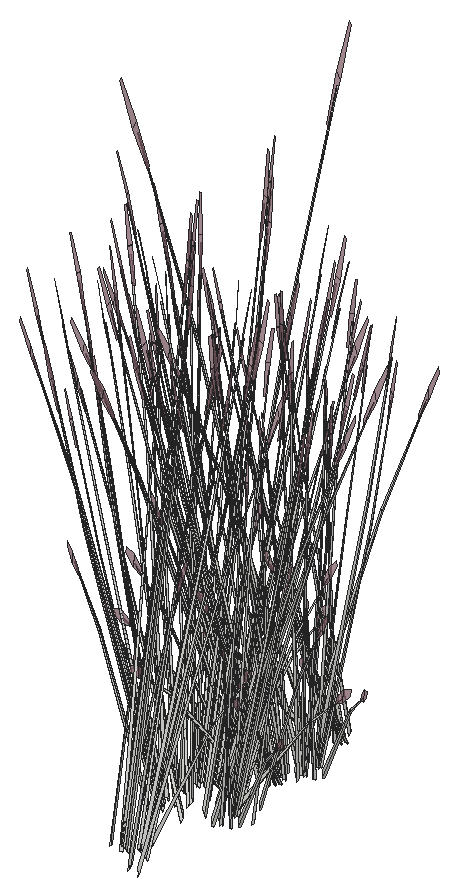
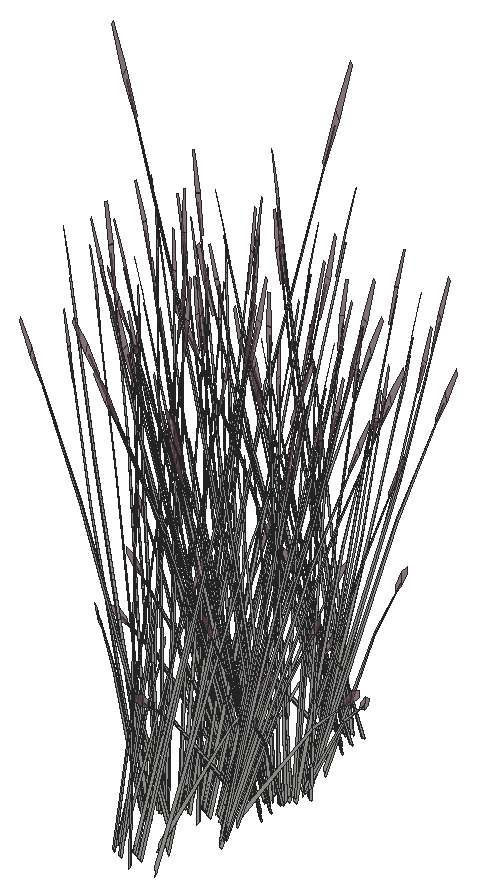
# SketchUp Ruby script. Lengths in inches.
U = 1.inch
M = Sketchup.active_model
def pt(a) = Geom::Point3d.new(a.map { |v| v * U })
def face(e, loops, mat)
  f = e.add_face(loops[0].map { |a| pt(a) })
  loops[1..].each { |l| e.add_face(l.map { |a| pt(a) }).erase! }
  f.material = f.back_material = mat if mat
  f
end
# faces: each face lists its corners as indices into pts; further lists are holes
def faces(e, pts, list, mat = nil) = list.each { |f| face(e, (f[0].is_a?(Array) ? f : [f]).map { |l| l.map { |i| pts[i] } }, mat) }
# xy, xz, yz: faces in a plane at the given z, y or x. An outline is a flat list of corners, or four numbers for a rectangle; further outlines are holes
def ring(l) = l.size == 4 ? [[l[0], l[1]], [l[2], l[1]], [l[2], l[3]], [l[0], l[3]]] : l.each_slice(2).to_a
def flat(e, list, mat, &to3) = list.each { |f| face(e, (f[0].is_a?(Array) ? f : [f]).map { |l| ring(l).map { |u, v| to3.(u, v) } }, mat) }
def xy(e, z, list, mat = nil) = flat(e, list, mat) { |x, y| [x, y, z] }
def xz(e, y, list, mat = nil) = flat(e, list, mat) { |x, z| [x, y, z] }
def yz(e, x, list, mat = nil) = flat(e, list, mat) { |y, z| [x, y, z] }
def lines(e, pts, list) = list.each { |a, b| e.add_line(pt(pts[a]), pt(pts[b])) }
# prism: a flat outline (further loops are holes) pulled along v
def prism(e, loops, v, mat = nil)
  f = face(e, loops, mat); d = Geom::Vector3d.new(v.map { |x| x * U })
  f.pushpull(f.normal.samedirection?(d) ? d.length : -d.length)
end
def box(e, o, s, mat = nil) = prism(e, [[o, [o[0] + s[0], o[1], o[2]], [o[0] + s[0], o[1] + s[1], o[2]], [o[0], o[1] + s[1], o[2]]]], [0, 0, s[2]], mat)
def at(x, y, z, deg = 0) = Geom::Transformation.translation(pt([x, y, z])) * Geom::Transformation.rotation(ORIGIN, Z_AXIS, deg.degrees)
def axes(o, x, y, z) = Geom::Transformation.new([*x, 0, *y, 0, *z, 0, *pt(o).to_a, 1])
def part(name) = M.definitions.add(name)
# library, detail: a bought-in or finely detailed component or shape, given as its bounding box
def library(name, o, s) = part(name).tap { |d| box(d.entities, o, s) }
def detail(e, o, s) = box(e.add_group.entities, o, s)
def put(e, d, t, mat = nil) = e.add_instance(d, t).tap { |i| i.material = mat if mat }
def group(e, t, mat = nil) = e.add_group.tap { |g| g.transformation = t; g.material = mat if mat }.entities
root = M.entities
M.materials.add("LightPink_Translucent").color = [144, 107, 117]
M.materials["LightPink_Translucent"].alpha = 0.75
c1 = part("blade")
p = [[2.15,0.21,22],[0,0.17,0],[0.09,0.45,0],[2.18,0.31,22],[2.29,0.31,22],[0.38,0.45,0],
  [2.48,0.24,33],[2.49,0.24,33],[2.48,0.22,33]]
faces(c1.entities,p,[[0,1,2,3],[4,5,2,3],[6,3,4,7],[8,0,3,6]])
c2 = part("seeds")
p = [[0.3,-0.1,1.38],[-0.01,-0.03,1.59],[-0.01,-0.03,0.03],[0.14,-0.07,-0.07],[0.29,-0.03,3],[0.15,0.01,3.11]]
faces(c2.entities,p,[[0,1,2,3],[1,0,4,5]],"LightPink_Translucent")
c3 = part("blade with seeds")
put(c3.entities,c1,at(0,0,0))
put(c3.entities,c2,axes([2.4,0.25,30.99],[1.5799,-0.05474,1.17369],[-0.12525,1.92788,0.29478],[-0.07173,-0.02425,1.56792]))
put(root,c3,axes([429.37,403.85,153.98],[-0.05353,-0.00358,1.49853],[-0.22227,-0.38383,-0.1416],[0.08926,-0.1262,0.26519]))
put(root,c3,axes([427.31,399,154],[-0.30197,0.1603,0.05432],[-0.1478,-0.29231,0.42765],[0.02916,0.12885,0.65209]))
put(root,c3,axes([426.5,398.62,153.82],[-0.27728,0.24833,-0.29918],[-0.26248,-0.28355,0.38624],[-0.03994,0.14407,0.73904]))
put(root,c3,axes([425.54,398.54,153.98],[-0.01019,0.09334,1.47793],[0.28908,0.3247,-0.23373],[-0.07568,0.15355,0.11853]))
put(root,c3,axes([426.47,398.33,154.56],[0.45039,0.02337,-0.11403],[-0.01231,0.44247,-0.63292],[-0.03129,0.17041,0.9617]))
put(root,c3,axes([427.3,398.83,154.25],[0.40102,-0.2196,-0.10273],[0.19707,0.38974,-0.57019],[0.05291,0.16424,0.8664]))
put(root,c3,axes([428.54,403.7,153.82],[0.35672,-0.06741,-0.29918],[0.09419,0.38534,0.38624],[0.10222,-0.1035,0.73904]))
put(root,c3,axes([425.19,403.06,154],[0.02064,-0.35866,0.05432],[0.3116,0.00983,0.42765],[-0.11936,-0.03753,0.65209]))
put(root,c3,axes([425.07,403.17,153.82],[-0.23317,-0.29531,-0.29918],[0.26625,-0.27955,0.38624],[-0.13527,-0.04253,0.73904]))
put(root,c3,axes([426.77,398.5,154.23],[0.29336,0.31691,-0.47917],[-0.3099,0.27755,-0.37115],[-0.04464,0.16102,0.91684]))
put(root,c3,axes([427.64,398.81,153.95],[0.40284,0.11824,-0.43168],[-0.13808,0.40538,-0.33437],[0.03694,0.16321,0.82598]))
put(root,c3,axes([427.87,397.97,153.27],[-0.09368,-0.15143,1.44779],[0.43286,-0.12749,0.11706],[0.09783,0.23774,0.61892]))
put(root,c3,axes([427.46,399.06,153.82],[-0.12355,0.36271,-0.29918],[-0.36044,-0.10579,0.38624],[0.03305,0.14603,0.73904]))
put(root,c3,axes([426.68,398.36,154.51],[-0.01066,0.43628,-0.66621],[-0.44902,-0.0293,0.0804],[-0.04739,0.18483,0.94242]))
put(root,c3,axes([425.32,403.37,154.21],[-0.40965,-0.01136,-0.60019],[0.02751,-0.47821,0.07243],[-0.17355,-0.05047,0.84903]))
put(root,c3,axes([425.51,399.5,153.98],[0.04649,-0.02848,1.49853],[0.38427,0.18941,-0.1416],[-0.00903,0.15771,0.26519]))
put(root,c3,axes([427.11,398.05,153.27],[-0.01003,-0.18103,1.44779],[0.43473,0.12009,0.11706],[-0.02689,0.25798,0.61892]))
put(root,c3,axes([428.57,403.87,154],[0.28133,0.19836,0.05432],[-0.16379,0.28248,0.42765],[0.0902,-0.09132,0.65209]))
put(root,c3,axes([429.57,404.31,153.98],[0.05687,-0.07184,1.47793],[-0.07279,-0.44069,-0.23373],[0.14268,-0.08356,0.11853]))
put(root,c3,axes([427.5,398.73,154.21],[0.19559,0.38351,-0.60019],[-0.40262,0.21373,0.07243],[0.04574,0.1853,0.84903]))
put(root,c3,axes([424.76,402.59,153.98],[0.03038,0.04707,1.49853],[-0.14646,0.42312,-0.1416],[-0.14833,0.00306,0.26519]))
put(root,c3,axes([427.2,399.7,153.98],[0.05195,0.07595,1.47793],[0.41921,0.02984,-0.23373],[0.04216,0.1675,0.11853]))
put(root,c3,axes([425.18,403.47,153.95],[-0.29757,0.31243,-0.43168],[-0.2606,-0.33005,-0.33437],[-0.15119,-0.04754,0.82598]))
put(root,c3,axes([425.34,403.14,154.25],[-0.02194,0.47967,-0.10273],[-0.41546,-0.01311,-0.57019],[-0.16001,-0.03332,0.8664]))
put(root,c3,axes([428.45,404.98,154.25],[-0.20619,-0.42709,-0.10273],[0.36595,-0.20988,-0.57019],[0.15422,-0.05635,0.8664]))
put(root,c3,axes([428.43,404.61,153.95],[0.11102,-0.42903,-0.43168],[0.38064,0.14706,-0.33437],[0.15325,-0.03934,0.82598]))
put(root,c3,axes([426.53,398.97,152.84],[0.009,-0.24349,1.30391],[0.40497,0.12861,0.18019],[-0.03509,0.2595,0.61571]))
put(root,c3,axes([424.81,403.8,153.27],[0.16998,-0.01068,1.44779],[-0.11276,0.46299,0.11706],[-0.24224,-0.02864,0.61892]))
put(root,c3,axes([428.36,404.77,154.21],[0.3601,-0.20831,-0.60019],[0.20068,0.4288,0.07243],[0.17399,-0.04871,0.84903]))
put(root,c3,axes([424.71,404.04,154],[-0.15051,-0.3216,0.05432],[0.27447,-0.15741,0.42765],[-0.12099,0.03106,0.65209]))
put(root,c3,axes([428.66,404.81,153.82],[0.34057,0.13158,-0.29918],[-0.09933,0.38387,0.38624],[0.13712,-0.0352,0.73904]))
put(root,c3,axes([424.66,404.2,153.82],[-0.34057,-0.13158,-0.29918],[0.09933,-0.38387,0.38624],[-0.13712,0.0352,0.73904]))
put(root,c3,axes([427.74,404.33,153.27],[-0.16998,0.01068,1.44779],[0.11276,-0.46299,0.11706],[0.24224,0.02864,0.61892]))
put(root,c3,axes([428.61,404.97,154],[0.15051,0.3216,0.05432],[-0.27447,0.15741,0.42765],[0.12099,-0.03106,0.65209]))
put(root,c3,axes([425.9,409.13,153.27],[0.09368,0.15143,1.44779],[-0.43286,0.12749,0.11706],[-0.09783,-0.23774,0.61892]))
put(root,c3,axes([426.62,408.13,153.98],[-0.06268,-0.06613,1.47793],[-0.4183,0.04193,-0.23373],[-0.06676,-0.15817,0.11853]))
put(root,c3,axes([425.7,404.13,152.82],[0.11649,-0.06823,1.49584],[0.04017,0.47639,0.11706],[-0.25231,0.06321,0.53462]))
put(root,c3,axes([427.06,409.25,154.21],[-0.19559,-0.38351,-0.60019],[0.40262,-0.21373,0.07243],[-0.04574,-0.1853,0.84903]))
put(root,c3,axes([429.27,406.25,153.98],[-0.03706,-0.04129,1.49853],[0.08106,-0.44261,-0.1416],[0.14596,-0.02828,0.26519]))
put(root,c3,axes([427.87,409.62,154.21],[0.01066,-0.43628,-0.60019],[0.44902,0.0293,0.07243],[0.04739,-0.18483,0.84903]))
put(root,c3,axes([424.45,404.45,153.98],[-0.06692,0.06124,1.47793],[0.00569,0.44742,-0.23373],[-0.15339,0.05818,0.11853]))
put(root,c3,axes([424.89,404.39,153.95],[-0.11102,0.42903,-0.43168],[-0.38064,-0.14706,-0.33437],[-0.15325,0.03934,0.82598]))
put(root,c3,axes([424.875,404.03,154.25],[0.20619,0.42709,-0.10273],[-0.36595,0.20988,-0.57019],[-0.15422,0.05635,0.8664]))
put(root,c3,axes([428.95,405.88,153.32],[-0.07843,-0.39649,-0.0295],[0.37072,-0.09115,-0.13375],[0.07742,0.02514,0.44114]))
put(root,c3,axes([428.5,408.9375,153.98],[-0.00396,-0.09387,1.47793],[-0.33411,-0.2713,-0.23373],[0.05166,-0.16446,0.11853]))
put(root,c3,axes([427.09,408.92,153.82],[0.12355,-0.36271,-0.29918],[0.36044,0.10579,0.38624],[-0.03305,-0.14603,0.73904]))
put(root,c3,axes([427.37,409.4,153.27],[-0.0763,0.16212,1.44779],[-0.3201,-0.3355,0.11706],[0.1444,-0.2091,0.61892]))
put(root,c3,axes([427.98,405.87,154.25],[0.02194,-0.47967,-0.10273],[0.41546,0.01311,-0.57019],[0.16001,0.03332,0.8664]))
put(root,c3,axes([428.41,408.6,153.98],[-0.04162,0.03603,1.49853],[-0.40776,-0.12155,-0.1416],[-0.01476,-0.15722,0.26519]))
put(root,c3,axes([426.91,409.17,153.95],[-0.40284,-0.11824,-0.43168],[0.13808,-0.40538,-0.33437],[-0.03694,-0.16321,0.82598]))
put(root,c3,axes([427.78,409.48,153.95],[-0.29336,-0.31691,-0.43168],[0.3099,-0.27755,-0.33437],[0.04464,-0.16102,0.82598]))
put(root,c3,axes([426.1875,407.91,153.98],[-0.00765,0.05653,1.49853],[-0.37706,0.20517,-0.1416],[-0.11096,-0.10488,0.26519]))
put(root,c3,axes([428.35,405.58,153.98],[0.08791,-0.00798,1.47793],[0.24113,-0.36643,-0.23373],[0.15637,0.04837,0.11853]))
put(root,c3,axes([427.25,409.15,154.25],[-0.40102,0.2196,-0.10273],[-0.19707,-0.38974,-0.57019],[-0.05291,-0.16424,0.8664]))
put(root,c3,axes([428.09,409.64,154.25],[-0.45039,-0.02337,-0.10273],[0.01231,-0.44247,-0.57019],[0.03129,-0.17041,0.8664]))
put(root,c3,axes([424.75,405.14,154],[-0.28133,-0.19836,0.05432],[0.16379,-0.28248,0.42765],[-0.0902,0.09132,0.65209]))
put(root,c3,axes([428.06,409.36,153.82],[0.27728,-0.24833,-0.29918],[0.26248,0.28355,0.38624],[0.03994,-0.14407,0.73904]))
put(root,c3,axes([424.88,404.61,153.27],[0.14219,-0.09977,1.44779],[0.11971,0.461,0.11706],[-0.22323,0.10419,0.61892]))
put(root,c3,axes([427.25,408.97,154],[0.30197,-0.1603,0.05432],[0.1478,0.29231,0.42765],[-0.02916,-0.12885,0.65209]))
put(root,c3,axes([426.17,409.35,154.21],[-0.34944,-0.22798,-0.60019],[0.24834,-0.39949,0.07243],[-0.1266,-0.13612,0.84903]))
put(root,c3,axes([426.05,409.05,153.82],[-0.06329,-0.37991,-0.29918],[0.36182,-0.10032,0.38624],[-0.09718,-0.10887,0.73904]))
put(root,c3,axes([428.01,405.64,154.21],[0.40965,0.01136,-0.60019],[-0.02751,0.47821,0.07243],[0.17355,0.05047,0.84903]))
put(root,c3,axes([426.21,409.02,154],[0.18625,-0.29962,0.05432],[0.26523,0.17444,0.42765],[-0.08575,-0.09606,0.65209]))
put(root,c3,axes([423.7,404.9,153.98],[0.0523,0.01265,1.49853],[0.16179,0.41674,-0.1416],[-0.10706,0.10938,0.26519]))
put(root,c3,axes([425.28,409.6,153.27],[0.15222,0.08126,1.44779],[-0.31502,0.34091,0.11706],[-0.19634,-0.15379,0.61892]))
put(root,c3,axes([428.25,405.83,153.82],[0.23317,0.29531,-0.29918],[-0.26625,0.27955,0.38624],[0.13527,0.04253,0.73904]))
put(root,c3,axes([428.13,405.95,154],[-0.02064,0.35866,0.05432],[-0.3116,-0.00983,0.42765],[0.11936,0.03753,0.65209]))
put(root,c3,axes([424.78,405.3,153.82],[-0.35672,0.06741,-0.29918],[-0.09419,-0.38534,0.38624],[-0.10222,0.1035,0.73904]))
put(root,c3,axes([426.01,409.37,153.95],[-0.40438,0.11212,-0.43168],[-0.07074,-0.4246,-0.33437],[-0.10862,-0.12168,0.82598]))
put(root,c3,axes([426.29,408.99,154.59],[-0.2735,0.45217,-0.11506],[-0.39608,-0.2605,-0.63862],[-0.13768,-0.12775,0.97037]))
put(root,c3,axes([428.16,409.49,154],[0.33677,0.02198,0.05432],[-0.00923,0.33185,0.42765],[0.03524,-0.12712,0.65209]))
put(root,c3,axes([428.4,410.38,154.21],[0.21406,-0.37215,-0.60019],[0.37511,0.26448,0.07243],[0.12781,-0.13483,0.84903]))
put(root,c3,axes([428.39,410.21,153.95],[-0.10528,-0.43067,-0.43168],[0.39868,-0.07534,-0.33437],[0.11425,-0.11568,0.82598]))
put(root,c3,axes([427.41,405.08,153.27],[-0.15222,-0.08126,1.44779],[0.31502,-0.34091,0.11706],[0.19634,0.15379,0.61892]))
put(root,c3,axes([425.25,408.86,153.98],[-0.08817,-0.00333,1.47793],[-0.28072,0.33293,-0.23373],[-0.14978,-0.06803,0.11853]))
put(root,c3,axes([428.58,410.51,154.25],[-0.37908,-0.26007,-0.10273],[0.21839,-0.37663,-0.57019],[0.1071,-0.13092,0.8664]))
put(root,c3,axes([427.44,404.01,153.78],[-0.35411,-0.24507,1.16821],[0.37391,-0.38156,0.50405],[0.11425,0.22994,1.12919]))
put(root,c3,axes([424.89,405.04,154.25],[0.37908,0.26007,-0.10273],[-0.21839,0.37663,-0.57019],[-0.1071,0.13092,0.8664]))
put(root,c3,axes([427.01,411.93,152.81],[0.35414,0.19019,1.27785],[-0.34693,0.40974,0.50532],[-0.1554,-0.24285,1.07126]))
put(root,c3,axes([427.17,406.39,154.25],[0.2442,-0.40372,-0.10273],[0.35364,0.23259,-0.57019],[0.12293,0.11406,0.8664]))
put(root,c3,axes([425.4,404.92,153.27],[0.10236,-0.14492,1.44779],[0.25844,0.39118,0.11706],[-0.17726,0.17814,0.61892]))
put(root,c3,axes([429.51,410.4,153.98],[-0.05353,-0.00358,1.49853],[-0.22227,-0.38383,-0.1416],[0.08926,-0.1262,0.26519]))
put(root,c3,axes([425.08,405.35,153.95],[0.10528,0.43067,-0.43168],[-0.39868,0.07534,-0.33437],[-0.11425,0.11568,0.82598]))
put(root,c3,axes([426.85,406.72,153.98],[0.00121,-0.0571,1.49853],[0.35119,-0.25193,-0.1416],[0.12199,0.08992,0.26519]))
put(root,c3,axes([425.31,406.07,154],[-0.33677,-0.02198,0.05432],[0.00923,-0.33185,0.42765],[-0.03524,0.12712,0.65209]))
put(root,c3,axes([427.46,406.1875,153.95],[0.40438,-0.11212,-0.43168],[0.07074,0.4246,-0.33437],[0.10862,0.12168,0.82598]))
put(root,c3,axes([428.68,410.25,153.82],[0.35672,-0.06741,-0.29918],[0.09419,0.38534,0.38624],[0.10222,-0.1035,0.73904]))
put(root,c3,axes([425.34,409.61,154],[0.02064,-0.35866,0.05432],[0.3116,0.00983,0.42765],[-0.11936,-0.03753,0.65209]))
put(root,c3,axes([425.22,409.72,153.82],[-0.23317,-0.29531,-0.29918],[0.26625,-0.27955,0.38624],[-0.13527,-0.04253,0.73904]))
put(root,c3,axes([427.26,406.54,154],[-0.18625,0.29962,0.05432],[-0.26523,-0.17444,0.42765],[0.08575,0.09606,0.65209]))
put(root,c3,axes([425.46,409.92,154.21],[-0.40965,-0.01136,-0.60019],[0.02751,-0.47821,0.07243],[-0.17355,-0.05047,0.84903]))
put(root,c3,axes([425.32,405.28,153.27],[0.0763,-0.16212,1.44779],[0.3201,0.3355,0.11706],[-0.1444,0.2091,0.61892]))
put(root,c3,axes([426.22,406.58,154],[-0.30197,0.1603,0.05432],[-0.1478,-0.29231,0.42765],[0.02916,0.12885,0.65209]))
put(root,c3,axes([425.41,406.2,153.82],[-0.27728,0.24833,-0.29918],[-0.26248,-0.28355,0.38624],[-0.03994,0.14407,0.73904]))
put(root,c3,axes([424.46,406.12,153.98],[-0.01019,0.09334,1.47793],[0.28908,0.3247,-0.23373],[-0.07568,0.15355,0.11853]))
put(root,c3,axes([428.72,410.42,154],[0.28133,0.19836,0.05432],[-0.16379,0.28248,0.42765],[0.0902,-0.09132,0.65209]))
put(root,c3,axes([425.38,405.91,154.56],[0.45039,0.02337,-0.11403],[-0.01231,0.44247,-0.63292],[-0.03129,0.17041,0.9617]))
put(root,c3,axes([426.21,406.4,154.25],[0.40102,-0.2196,-0.10273],[0.19707,0.38974,-0.57019],[0.05291,0.16424,0.8664]))
put(root,c3,axes([429.71,410.86,153.98],[0.05687,-0.07184,1.47793],[-0.07279,-0.44069,-0.23373],[0.14268,-0.08356,0.11853]))
put(root,c3,axes([424.91,409.14,153.98],[0.03038,0.04707,1.49853],[-0.14646,0.42312,-0.1416],[-0.14833,0.00306,0.26519]))
put(root,c3,axes([425.6875,406.08,154.23],[0.29336,0.31691,-0.47917],[-0.3099,0.27755,-0.37115],[-0.04464,0.16102,0.91684]))
put(root,c3,axes([425.33,410.01,153.95],[-0.29757,0.31243,-0.43168],[-0.2606,-0.33005,-0.33437],[-0.15119,-0.04754,0.82598]))
put(root,c3,axes([426.56,406.39,153.95],[0.40284,0.11824,-0.43168],[-0.13808,0.40538,-0.33437],[0.03694,0.16321,0.82598]))
put(root,c3,axes([426.79,405.55,153.27],[-0.09368,-0.15143,1.44779],[0.43286,-0.12749,0.11706],[0.09783,0.23774,0.61892]))
put(root,c3,axes([425.48,409.6875,154.25],[-0.02194,0.47967,-0.10273],[-0.41546,-0.01311,-0.57019],[-0.16001,-0.03332,0.8664]))
put(root,c3,axes([426.375,406.63,153.82],[-0.12355,0.36271,-0.29918],[-0.36044,-0.10579,0.38624],[0.03305,0.14603,0.73904]))
put(root,c3,axes([428.59,411.53,154.25],[-0.20619,-0.42709,-0.10273],[0.36595,-0.20988,-0.57019],[0.15422,-0.05635,0.8664]))
put(root,c3,axes([428.57,411.16,153.95],[0.11102,-0.42903,-0.43168],[0.38064,0.14706,-0.33437],[0.15325,-0.03934,0.82598]))
put(root,c3,axes([425.6,405.93,154.51],[-0.01066,0.43628,-0.66621],[-0.44902,-0.0293,0.0804],[-0.04739,0.18483,0.94242]))
put(root,c3,axes([424.95,410.35,153.27],[0.16998,-0.01068,1.44779],[-0.11276,0.46299,0.11706],[-0.24224,-0.02864,0.61892]))
put(root,c3,axes([424.42,407.08,153.98],[0.04649,-0.02848,1.49853],[0.38427,0.18941,-0.1416],[-0.00903,0.15771,0.26519]))
put(root,c3,axes([426.02,405.625,153.27],[-0.01003,-0.18103,1.44779],[0.43473,0.12009,0.11706],[-0.02689,0.25798,0.61892]))
put(root,c3,axes([428.5,411.32,154.21],[0.3601,-0.20831,-0.60019],[0.20068,0.4288,0.07243],[0.17399,-0.04871,0.84903]))
put(root,c3,axes([426.41,406.31,154.21],[0.19559,0.38351,-0.60019],[-0.40262,0.21373,0.07243],[0.04574,0.1853,0.84903]))
put(root,c3,axes([426.12,407.28,153.98],[0.05195,0.07595,1.47793],[0.41921,0.02984,-0.23373],[0.04216,0.1675,0.11853]))
put(root,c3,axes([425.83,414.51,153.27],[0.09368,0.15143,1.44779],[-0.43286,0.12749,0.11706],[-0.09783,-0.23774,0.61892]))
put(root,c3,axes([426.55,413.51,153.98],[-0.06268,-0.06613,1.47793],[-0.4183,0.04193,-0.23373],[-0.06676,-0.15817,0.11853]))
put(root,c3,axes([424.85,410.58,154],[-0.15051,-0.3216,0.05432],[0.27447,-0.15741,0.42765],[-0.12099,0.03106,0.65209]))
put(root,c3,axes([426.99,414.63,154.21],[-0.19559,-0.38351,-0.60019],[0.40262,-0.21373,0.07243],[-0.04574,-0.1853,0.84903]))
put(root,c3,axes([425.45,406.55,152.84],[0.009,-0.24349,1.30391],[0.40497,0.12861,0.18019],[-0.03509,0.2595,0.61571]))
put(root,c3,axes([428.81,411.36,153.82],[0.34057,0.13158,-0.29918],[-0.09933,0.38387,0.38624],[0.13712,-0.0352,0.73904]))
put(root,c3,axes([427.8,415,154.21],[0.01066,-0.43628,-0.60019],[0.44902,0.0293,0.07243],[0.04739,-0.18483,0.84903]))
put(root,c3,axes([424.8,410.75,153.82],[-0.34057,-0.13158,-0.29918],[0.09933,-0.38387,0.38624],[-0.13712,0.0352,0.73904]))
put(root,c3,axes([428.43,414.32,153.98],[-0.00396,-0.09387,1.47793],[-0.33411,-0.2713,-0.23373],[0.05166,-0.16446,0.11853]))
put(root,c3,axes([427.02,414.3,153.82],[0.12355,-0.36271,-0.29918],[0.36044,0.10579,0.38624],[-0.03305,-0.14603,0.73904]))
put(root,c3,axes([427.3,414.78,153.27],[-0.0763,0.16212,1.44779],[-0.3201,-0.3355,0.11706],[0.1444,-0.2091,0.61892]))
put(root,c3,axes([428.34,413.98,153.98],[-0.04162,0.03603,1.49853],[-0.40776,-0.12155,-0.1416],[-0.01476,-0.15722,0.26519]))
put(root,c3,axes([427.88,410.88,153.27],[-0.16998,0.01068,1.44779],[0.11276,-0.46299,0.11706],[0.24224,0.02864,0.61892]))
put(root,c3,axes([426.84,414.55,153.95],[-0.40284,-0.11824,-0.43168],[0.13808,-0.40538,-0.33437],[-0.03694,-0.16321,0.82598]))
put(root,c3,axes([427.71,414.86,153.95],[-0.29336,-0.31691,-0.43168],[0.3099,-0.27755,-0.33437],[0.04464,-0.16102,0.82598]))
